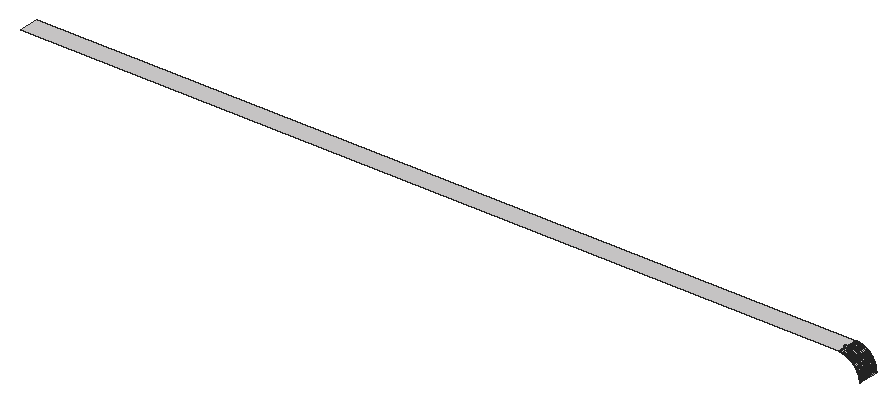
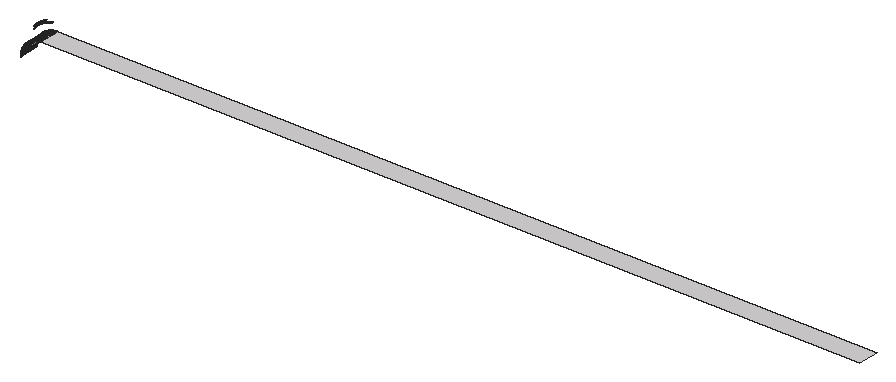
# SketchUp Ruby script. Lengths in inches.
U = 1.inch
M = Sketchup.active_model
def pt(a) = Geom::Point3d.new(a.map { |v| v * U })
def face(e, loops, mat)
  f = e.add_face(loops[0].map { |a| pt(a) })
  loops[1..].each { |l| e.add_face(l.map { |a| pt(a) }).erase! }
  f.material = f.back_material = mat if mat
  f
end
# faces: each face lists its corners as indices into pts; further lists are holes
def faces(e, pts, list, mat = nil) = list.each { |f| face(e, (f[0].is_a?(Array) ? f : [f]).map { |l| l.map { |i| pts[i] } }, mat) }
# xy, xz, yz: faces in a plane at the given z, y or x. An outline is a flat list of corners, or four numbers for a rectangle; further outlines are holes
def ring(l) = l.size == 4 ? [[l[0], l[1]], [l[2], l[1]], [l[2], l[3]], [l[0], l[3]]] : l.each_slice(2).to_a
def flat(e, list, mat, &to3) = list.each { |f| face(e, (f[0].is_a?(Array) ? f : [f]).map { |l| ring(l).map { |u, v| to3.(u, v) } }, mat) }
def xy(e, z, list, mat = nil) = flat(e, list, mat) { |x, y| [x, y, z] }
def xz(e, y, list, mat = nil) = flat(e, list, mat) { |x, z| [x, y, z] }
def yz(e, x, list, mat = nil) = flat(e, list, mat) { |y, z| [x, y, z] }
def lines(e, pts, list) = list.each { |a, b| e.add_line(pt(pts[a]), pt(pts[b])) }
# prism: a flat outline (further loops are holes) pulled along v
def prism(e, loops, v, mat = nil)
  f = face(e, loops, mat); d = Geom::Vector3d.new(v.map { |x| x * U })
  f.pushpull(f.normal.samedirection?(d) ? d.length : -d.length)
end
def box(e, o, s, mat = nil) = prism(e, [[o, [o[0] + s[0], o[1], o[2]], [o[0] + s[0], o[1] + s[1], o[2]], [o[0], o[1] + s[1], o[2]]]], [0, 0, s[2]], mat)
def at(x, y, z, deg = 0) = Geom::Transformation.translation(pt([x, y, z])) * Geom::Transformation.rotation(ORIGIN, Z_AXIS, deg.degrees)
def axes(o, x, y, z) = Geom::Transformation.new([*x, 0, *y, 0, *z, 0, *pt(o).to_a, 1])
def part(name) = M.definitions.add(name)
# library, detail: a bought-in or finely detailed component or shape, given as its bounding box
def library(name, o, s) = part(name).tap { |d| box(d.entities, o, s) }
def detail(e, o, s) = box(e.add_group.entities, o, s)
def put(e, d, t, mat = nil) = e.add_instance(d, t).tap { |i| i.material = mat if mat }
def group(e, t, mat = nil) = e.add_group.tap { |g| g.transformation = t; g.material = mat if mat }.entities
root = M.entities
M.materials.add("[Quartz Light Brown]").color = [215, 212, 212]
xy(root,95.96,[[504.94,38,505.04,50]],"[Quartz Light Brown]")
xy(root,95.98,[[504.66,38,504.75,50]],"[Quartz Light Brown]")
xy(root,95.99,[[504.375,38,504.47,50],[504.47,38,504.57,50]],"[Quartz Light Brown]")
xy(root,96,[[36,38,504,50],[504,38,504.09,50],[504.09,38,504.1875,50],[504.1875,38,504.28,50]],"[Quartz Light Brown]")
yz(root,515.96,[[38,84.94,50,85.04]],"[Quartz Light Brown]")
yz(root,515.98,[[38,84.66,50,84.75]],"[Quartz Light Brown]")
yz(root,515.99,[[38,84.375,50,84.47],[38,84.47,50,84.57]],"[Quartz Light Brown]")
yz(root,516,[[38,84,50,84.09],[38,84.09,50,84.1875],[38,84.1875,50,84.28]],"[Quartz Light Brown]")
p = [[516,38,84.28],[515.99,38,84.375],[515.99,50,84.375],[516,50,84.28],[515.99,38,84.57],[515.98,38,84.66],
  [515.98,50,84.66],[515.99,50,84.57],[515.97,38,84.85],[515.96,38,84.94],[515.96,50,84.94],[515.97,50,84.85],
  [515.98,38,84.75],[515.98,50,84.75],[515.96,38,85.04],[515.95,38,85.13],[515.95,50,85.13],[515.96,50,85.04],
  [515.9375,38,85.22],[515.9375,50,85.22],[515.93,38,85.32],[515.93,50,85.32],[515.92,38,85.41],[515.92,50,85.41],
  [515.91,38,85.5],[515.91,50,85.5],[515.89,38,85.6],[515.89,50,85.6],[515.88,38,85.69],[515.88,50,85.69],
  [515.87,38,85.78],[515.87,50,85.78],[515.85,38,85.88],[515.85,50,85.88],[515.84,38,85.97],[515.84,50,85.97],
  [515.82,38,86.0625],[515.82,50,86.0625],[515.8,38,86.16],[515.8,50,86.16],[515.79,38,86.25],[515.77,38,86.34],
  [515.77,50,86.34],[515.79,50,86.25],[515.75,38,86.43],[515.75,50,86.43],[515.73,38,86.53],[515.73,50,86.53],
  [515.71,38,86.62],[515.71,50,86.62],[515.69,38,86.71],[515.69,50,86.71],[515.67,38,86.8],[515.67,50,86.8],
  [515.65,38,86.89],[515.65,50,86.89],[515.62,38,86.98],[515.62,50,86.98],[515.6,38,87.08],[515.6,50,87.08],
  [515.57,38,87.17],[515.57,50,87.17],[515.55,38,87.26],[515.55,50,87.26],[515.52,38,87.35],[515.5,38,87.4375],
  [515.5,50,87.4375],[515.52,50,87.35],[515.47,38,87.53],[515.47,50,87.53],[515.44,38,87.62],[515.44,50,87.62],
  [515.41,38,87.71],[515.41,50,87.71],[515.38,38,87.8],[515.38,50,87.8],[515.35,38,87.89],[515.35,50,87.89],
  [515.32,38,87.98],[515.32,50,87.98],[515.29,38,88.06],[515.29,50,88.06],[515.26,38,88.15],[515.26,50,88.15],
  [515.23,38,88.24],[515.19,38,88.33],[515.19,50,88.33],[515.23,50,88.24],[515.16,38,88.42],[515.16,50,88.42],
  [515.12,38,88.5],[515.12,50,88.5],[515.09,38,88.59],[515.09,50,88.59],[515.05,38,88.68],[515.05,50,88.68],
  [515.01,38,88.77],[515.01,50,88.77],[514.98,38,88.85],[514.98,50,88.85],[514.9375,38,88.9375],[514.9,38,89.02],
  [514.9,50,89.02],[514.9375,50,88.9375],[514.86,38,89.11],[514.86,50,89.11],[514.82,38,89.19],[514.82,50,89.19],
  [514.78,38,89.28],[514.78,50,89.28],[514.73,38,89.36],[514.73,50,89.36],[514.69,38,89.45],[514.65,38,89.53],
  [514.65,50,89.53],[514.69,50,89.45],[514.61,38,89.62],[514.61,50,89.62],[514.5625,38,89.7],[514.5625,50,89.7],
  [514.52,38,89.78],[514.52,50,89.78],[514.47,38,89.86],[514.47,50,89.86],[514.42,38,89.95],[514.375,38,90.03],
  [514.375,50,90.03],[514.42,50,89.95],[514.33,38,90.11],[514.33,50,90.11],[514.28,38,90.1875],[514.28,50,90.1875],
  [514.23,38,90.27],[514.23,50,90.27],[514.18,38,90.35],[514.18,50,90.35],[514.13,38,90.43],[514.08,38,90.51],
  [514.08,50,90.51],[514.13,50,90.43],[514.03,38,90.59],[514.03,50,90.59],[513.98,38,90.67],[513.98,50,90.67],
  [513.92,38,90.75],[513.87,38,90.82],[513.87,50,90.82],[513.92,50,90.75],[513.82,38,90.9],[513.82,50,90.9],
  [513.76,38,90.98],[513.76,50,90.98],[513.71,38,91.05],[513.71,50,91.05],[513.65,38,91.13],[513.6,38,91.21],
  [513.6,50,91.21],[513.65,50,91.13],[513.54,38,91.28],[513.54,50,91.28],[513.48,38,91.35],[513.48,50,91.35],
  [513.42,38,91.43],[513.37,38,91.5],[513.37,50,91.5],[513.42,50,91.43],[513.31,38,91.58],[513.31,50,91.58],
  [513.25,38,91.65],[513.1875,38,91.72],[513.1875,50,91.72],[513.25,50,91.65],[513.125,38,91.79],[513.125,50,91.79],
  [513.0625,38,91.86],[513.0625,50,91.86],[513,38,91.9375],[512.9375,38,92.01],[512.9375,50,92.01],[513,50,91.9375],
  [512.875,38,92.08],[512.875,50,92.08],[512.8125,38,92.15],[512.75,38,92.21],[512.75,50,92.21],[512.8125,50,92.15],
  [512.68,38,92.28],[512.68,50,92.28],[512.62,38,92.35],[512.62,50,92.35],[512.55,38,92.42],[512.49,38,92.49],
  [512.49,50,92.49],[512.55,50,92.42],[512.42,38,92.55],[512.42,50,92.55],[512.35,38,92.62],[512.28,38,92.68],
  [512.28,50,92.68],[512.35,50,92.62],[512.21,38,92.75],[512.15,38,92.8125],[512.15,50,92.8125],[512.21,50,92.75],
  [512.08,38,92.875],[512.08,50,92.875],[512.01,38,92.9375],[511.9375,38,93],[511.9375,50,93],[512.01,50,92.9375],
  [511.86,38,93.0625],[511.86,50,93.0625],[511.79,38,93.125],[511.72,38,93.1875],[511.72,50,93.1875],[511.79,50,93.125],
  [511.65,38,93.25],[511.58,38,93.31],[511.58,50,93.31],[511.65,50,93.25],[511.5,38,93.37],[511.5,50,93.37],
  [511.43,38,93.42],[511.35,38,93.48],[511.35,50,93.48],[511.43,50,93.42],[516.87,39,93.51],[516.87,38,93.51],
  [516.94,38,93.4],[516.94,39,93.4],[511.28,38,93.54],[511.21,38,93.6],[511.21,50,93.6],[511.28,50,93.54],
  [516.79,39,93.61],[516.79,38,93.61],[511.13,38,93.65],[511.13,50,93.65],[516.72,39,93.71],[516.72,38,93.71],
  [511.05,38,93.71],[510.98,38,93.76],[510.98,50,93.76],[511.05,50,93.71],[516.64,39,93.81],[516.64,38,93.81],
  [510.9,38,93.82],[510.82,38,93.87],[510.82,50,93.87],[510.9,50,93.82],[516.56,39,93.91],[516.56,38,93.91],
  [510.75,38,93.92],[510.67,38,93.98],[510.67,50,93.98],[510.75,50,93.92],[516.49,39,94],[516.49,38,94],
  [510.59,38,94.03],[510.51,38,94.08],[510.51,50,94.08],[510.59,50,94.03],[516.41,39,94.1],[516.41,38,94.1],
  [510.43,38,94.13],[510.35,38,94.18],[510.35,50,94.18],[510.43,50,94.13],[516.33,39,94.2],[516.33,38,94.2],
  [510.27,38,94.23],[510.1875,38,94.28],[510.1875,50,94.28],[510.27,50,94.23],[516.25,39,94.3],[516.25,38,94.3],
  [510.11,38,94.33],[510.03,38,94.375],[510.03,50,94.375],[510.11,50,94.33],[516.17,39,94.39],[516.17,38,94.39],
  [509.95,38,94.42],[509.86,38,94.47],[509.86,50,94.47],[509.95,50,94.42],[516.08,39,94.49],[516.08,38,94.49],
  [509.78,38,94.52],[509.7,38,94.5625],[509.7,50,94.5625],[509.78,50,94.52],[516,39,94.58],[516,38,94.58],
  [509.53,38,94.65],[509.45,38,94.69],[509.45,50,94.69],[509.53,50,94.65],[509.62,38,94.61],[509.62,50,94.61],
  [515.92,39,94.67],[515.92,38,94.67],[509.36,38,94.73],[509.28,38,94.78],[509.28,50,94.78],[509.36,50,94.73],
  [515.83,39,94.77],[515.83,38,94.77],[509.19,38,94.82],[509.11,38,94.86],[509.11,50,94.86],[509.19,50,94.82],
  [515.75,39,94.86],[515.75,38,94.86],[508.9375,38,94.9375],[508.85,38,94.98],[508.85,50,94.98],[508.9375,50,94.9375],
  [509.02,38,94.9],[509.02,50,94.9],[515.66,39,94.95],[515.66,38,94.95],[508.77,38,95.01],[508.68,38,95.05],
  [508.68,50,95.05],[508.77,50,95.01],[515.49,39,95.13],[515.49,38,95.13],[515.58,38,95.04],[515.58,39,95.04],
  [516.84,38,95.14],[516.84,39,95.14],[516.93,39,95.04],[516.93,38,95.04],[508.5,38,95.12],[508.42,38,95.16],
  [508.42,50,95.16],[508.5,50,95.12],[508.59,38,95.09],[508.59,50,95.09],[515.4,39,95.22],[515.4,38,95.22],
  [516.75,38,95.24],[516.75,39,95.24],[508.24,38,95.23],[508.15,38,95.26],[508.15,50,95.26],[508.24,50,95.23],
  [508.33,38,95.19],[508.33,50,95.19],[515.3125,39,95.3125],[515.3125,38,95.3125],[516.66,38,95.34],[516.66,39,95.34],
  [507.98,38,95.32],[507.89,38,95.35],[507.89,50,95.35],[507.98,50,95.32],[508.06,38,95.29],[508.06,50,95.29],
  [515.22,39,95.4],[515.22,38,95.4],[516.57,38,95.44],[516.57,39,95.44],[507.62,38,95.44],[507.53,38,95.47],
  [507.53,50,95.47],[507.62,50,95.44],[507.71,38,95.41],[507.71,50,95.41],[507.8,38,95.38],[507.8,50,95.38],
  [515.13,39,95.49],[515.13,38,95.49],[516.48,38,95.54],[516.48,39,95.54],[507.26,38,95.55],[507.17,38,95.57],
  [507.17,50,95.57],[507.26,50,95.55],[507.35,38,95.52],[507.35,50,95.52],[507.4375,38,95.5],[507.4375,50,95.5],
  [515.04,39,95.58],[515.04,38,95.58],[516.39,38,95.64],[516.39,39,95.64],[506.89,38,95.65],[506.8,38,95.67],
  [506.8,50,95.67],[506.89,50,95.65],[506.98,38,95.62],[506.98,50,95.62],[507.08,38,95.6],[507.08,50,95.6],
  [514.95,39,95.66],[514.95,38,95.66],[516.3,38,95.73],[516.3,39,95.73],[506.53,38,95.73],[506.43,38,95.75],
  [506.43,50,95.75],[506.53,50,95.73],[506.62,38,95.71],[506.62,50,95.71],[506.71,38,95.69],[506.71,50,95.69],
  [514.77,39,95.83],[514.77,38,95.83],[514.86,38,95.75],[514.86,39,95.75],[516.21,38,95.83],[516.21,39,95.83],
  [505.97,38,95.84],[505.88,38,95.85],[505.88,50,95.85],[505.97,50,95.84],[506.0625,38,95.82],[506.0625,50,95.82],
  [506.16,38,95.8],[506.16,50,95.8],[506.25,38,95.79],[506.25,50,95.79],[506.34,38,95.77],[506.34,50,95.77],
  [514.67,39,95.92],[514.67,38,95.92],[516.11,38,95.93],[516.11,39,95.93],[505.13,38,95.95],[505.04,38,95.96],
  [505.04,50,95.96],[505.13,50,95.95],[505.22,38,95.9375],[505.22,50,95.9375],[505.32,38,95.93],[505.32,50,95.93],
  [505.41,38,95.92],[505.41,50,95.92],[505.5,38,95.91],[505.5,50,95.91],[505.6,38,95.89],[505.6,50,95.89],
  [505.69,38,95.88],[505.69,50,95.88],[505.78,38,95.87],[505.78,50,95.87],[514.58,39,96],[514.58,38,96],
  [516.02,38,96.02],[516.02,39,96.02],[504.375,38,95.99],[504.28,38,96],[504.28,50,96],[504.375,50,95.99],
  [504.66,38,95.98],[504.57,38,95.99],[504.57,50,95.99],[504.66,50,95.98],[504.85,38,95.97],[504.75,38,95.98],
  [504.75,50,95.98],[504.85,50,95.97],[504.94,38,95.96],[504.94,50,95.96],[514.49,39,96.08],[514.49,38,96.08],
  [515.93,38,96.11],[515.93,39,96.11],[514.39,39,96.17],[514.39,38,96.17],[515.83,38,96.21],[515.83,39,96.21],
  [514.2,39,96.33],[514.2,38,96.33],[514.3,38,96.25],[514.3,39,96.25],[515.73,38,96.3],[515.73,39,96.3],
  [514.1,39,96.41],[514.1,38,96.41],[515.64,38,96.39],[515.64,39,96.39],[514,39,96.49],[514,38,96.49],
  [515.54,38,96.48],[515.54,39,96.48],[513.91,39,96.56],[513.91,38,96.56],[515.44,38,96.57],[515.44,39,96.57],
  [513.71,39,96.72],[513.71,38,96.72],[513.81,38,96.64],[513.81,39,96.64],[515.34,38,96.66],[515.34,39,96.66],
  [513.61,39,96.79],[513.61,38,96.79],[515.24,38,96.75],[515.24,39,96.75],[513.51,39,96.87],[513.51,38,96.87],
  [515.04,38,96.93],[515.04,39,96.93],[515.14,39,96.84],[515.14,38,96.84],[513.3,39,97.02],[513.3,38,97.02],
  [513.4,38,96.94],[513.4,39,96.94],[514.9375,38,97.01],[514.9375,39,97.01],[513.2,39,97.09],[513.2,38,97.09],
  [514.84,38,97.1],[514.84,39,97.1],[513.1,39,97.16],[513.1,38,97.16],[514.73,38,97.18],[514.73,39,97.18],
  [512.89,39,97.3],[512.89,38,97.3],[512.99,38,97.23],[512.99,39,97.23],[514.63,38,97.27],[514.63,39,97.27],
  [512.78,39,97.37],[512.78,38,97.37],[514.52,38,97.35],[514.52,39,97.35],[512.57,39,97.51],[512.57,38,97.51],
  [512.68,38,97.44],[512.68,39,97.44],[514.3125,38,97.51],[514.3125,39,97.51],[514.42,39,97.43],[514.42,38,97.43],
  [512.47,39,97.58],[512.47,38,97.58],[514.21,38,97.59],[514.21,39,97.59],[512.25,39,97.71],[512.25,38,97.71],
  [512.36,38,97.64],[512.36,39,97.64],[514.1,38,97.67],[514.1,39,97.67],[512.14,39,97.77],[512.14,38,97.77],
  [513.99,38,97.75],[513.99,39,97.75],[511.93,39,97.9],[511.93,38,97.9],[512.04,38,97.84],[512.04,39,97.84],
  [513.78,38,97.91],[513.78,39,97.91],[513.88,39,97.83],[513.88,38,97.83],[511.82,39,97.96],[511.82,38,97.96],
  [513.67,38,97.98],[513.67,39,97.98],[511.6,39,98.08],[511.6,38,98.08],[511.71,38,98.02],[511.71,39,98.02],
  [513.56,38,98.06],[513.56,39,98.06],[511.375,39,98.2],[511.375,38,98.2],[511.49,38,98.14],[511.49,39,98.14],
  [513.33,38,98.21],[513.33,39,98.21],[513.44,39,98.13],[513.44,38,98.13],[511.26,39,98.26],[511.26,38,98.26],
  [513.22,38,98.28],[513.22,39,98.28],[511.04,39,98.37],[511.04,38,98.37],[511.15,38,98.3125],[511.15,39,98.3125],
  [513.11,38,98.35],[513.11,39,98.35],[510.8125,39,98.48],[510.8125,38,98.48],[510.93,38,98.42],[510.93,39,98.42],
  [512.88,38,98.49],[512.88,39,98.49],[513,39,98.42],[513,38,98.42],[510.58,39,98.58],[510.58,38,98.58],
  [510.7,38,98.53],[510.7,39,98.53],[512.77,38,98.5625],[512.77,39,98.5625],[510.35,39,98.68],[510.35,38,98.68],
  [510.47,38,98.63],[510.47,39,98.63],[512.54,38,98.7],[512.54,39,98.7],[512.65,39,98.63],[512.65,38,98.63],
  [510.12,39,98.78],[510.12,38,98.78],[510.24,38,98.73],[510.24,39,98.73],[512.42,38,98.77],[512.42,39,98.77],
  [509.89,39,98.875],[509.89,38,98.875],[510.01,38,98.83],[510.01,39,98.83],[512.19,38,98.9],[512.19,39,98.9],
  [512.31,39,98.83],[512.31,38,98.83],[509.66,39,98.97],[509.66,38,98.97],[509.77,38,98.92],[509.77,39,98.92],
  [512.07,38,98.96],[512.07,39,98.96],[509.42,39,99.05],[509.42,38,99.05],[509.54,38,99.01],[509.54,39,99.01],
  [511.84,38,99.09],[511.84,39,99.09],[511.95,39,99.02],[511.95,38,99.02],[509.0625,39,99.18],[509.0625,38,99.18],
  [509.18,38,99.14],[509.18,39,99.14],[509.3,38,99.1],[509.3,39,99.1],[511.6,38,99.21],[511.6,39,99.21],
  [511.72,39,99.15],[511.72,38,99.15],[508.82,39,99.26],[508.82,38,99.26],[508.94,38,99.22],[508.94,39,99.22],
  [511.48,38,99.27],[511.48,39,99.27],[508.46,39,99.36],[508.46,38,99.36],[508.58,38,99.33],[508.58,39,99.33],
  [508.7,38,99.29],[508.7,39,99.29],[511.24,38,99.38],[511.24,39,99.38],[511.36,39,99.32],[511.36,38,99.32],
  [508.1,39,99.47],[508.1,38,99.47],[508.22,38,99.43],[508.22,39,99.43],[508.34,38,99.4],[508.34,39,99.4],
  [511,38,99.49],[511,39,99.49],[511.12,39,99.4375],[511.12,38,99.4375],[507.74,39,99.56],[507.74,38,99.56],
  [507.86,38,99.53],[507.86,39,99.53],[507.98,38,99.5],[507.98,39,99.5],[510.75,38,99.6],[510.75,39,99.6],
  [510.875,39,99.55],[510.875,38,99.55],[507.24,39,99.67],[507.24,38,99.67],[507.37,38,99.64],[507.37,39,99.64],
  [507.49,38,99.61],[507.49,39,99.61],[507.61,38,99.59],[507.61,39,99.59],[510.63,38,99.65],[510.63,39,99.65],
  [506.75,39,99.76],[506.75,38,99.76],[506.875,38,99.74],[506.875,39,99.74],[507,38,99.72],[507,39,99.72],
  [507.12,38,99.69],[507.12,39,99.69],[510.38,38,99.76],[510.38,39,99.76],[510.51,39,99.71],[510.51,38,99.71],
  [510.26,38,99.81],[510.26,39,99.81]]
faces(root,p,[[0,1,2,3],[4,5,6,7],[8,9,10,11],[12,8,11,13],[14,15,16,17],[15,18,19,16],[18,20,21,19],[20,22,23,21],
  [22,24,25,23],[24,26,27,25],[26,28,29,27],[28,30,31,29],[30,32,33,31],[32,34,35,33],[34,36,37,35],[36,38,39,37],
  [40,41,42,43],[38,40,43,39],[41,44,45,42],[44,46,47,45],[46,48,49,47],[48,50,51,49],[50,52,53,51],[52,54,55,53],
  [54,56,57,55],[56,58,59,57],[58,60,61,59],[60,62,63,61],[64,65,66,67],[62,64,67,63],[65,68,69,66],[68,70,71,69],
  [70,72,73,71],[72,74,75,73],[74,76,77,75],[76,78,79,77],[78,80,81,79],[80,82,83,81],[84,85,86,87],[82,84,87,83],
  [85,88,89,86],[88,90,91,89],[90,92,93,91],[92,94,95,93],[94,96,97,95],[96,98,99,97],[100,101,102,103],[98,100,103,99],
  [101,104,105,102],[104,106,107,105],[106,108,109,107],[108,110,111,109],[112,113,114,115],[110,112,115,111],[113,116,117,114],[116,118,119,117],
  [118,120,121,119],[120,122,123,121],[124,125,126,127],[122,124,127,123],[125,128,129,126],[128,130,131,129],[130,132,133,131],[132,134,135,133],
  [136,137,138,139],[134,136,139,135],[137,140,141,138],[140,142,143,141],[144,145,146,147],[142,144,147,143],[145,148,149,146],[148,150,151,149],
  [150,152,153,151],[154,155,156,157],[152,154,157,153],[155,158,159,156],[158,160,161,159],[162,163,164,165],[160,162,165,161],[163,166,167,164],
  [168,169,170,171],[166,168,171,167],[169,172,173,170],[172,174,175,173],[176,177,178,179],[174,176,179,175],[177,180,181,178],[182,183,184,185],
  [180,182,185,181],[183,186,187,184],[186,188,189,187],[190,191,192,193],[188,190,193,189],[191,194,195,192],[196,197,198,199],[194,196,199,195],
  [200,201,202,203],[197,200,203,198],[201,204,205,202],[206,207,208,209],[204,206,209,205],[207,210,211,208],[212,213,214,215],[210,212,215,211],
  [216,217,218,219],[213,216,219,214],[217,220,221,218],[222,223,224,225],[220,222,225,221],[226,227,228,229],[230,231,232,233],[223,230,233,224],
  [234,235,227,226],[231,236,237,232],[238,239,235,234],[240,241,242,243],[236,240,243,237],[244,245,239,238],[246,247,248,249],[241,246,249,242],
  [250,251,245,244],[252,253,254,255],[247,252,255,248],[256,257,251,250],[258,259,260,261],[253,258,261,254],[262,263,257,256],[264,265,266,267],
  [259,264,267,260],[268,269,263,262],[270,271,272,273],[265,270,273,266],[274,275,269,268],[276,277,278,279],[271,276,279,272],[280,281,275,274],
  [282,283,284,285],[277,282,285,278],[286,287,281,280],[288,289,290,291],[283,288,291,284],[292,293,287,286],[294,295,296,297],[298,294,297,299],
  [289,298,299,290],[300,301,293,292],[302,303,304,305],[295,302,305,296],[306,307,301,300],[308,309,310,311],[303,308,311,304],[312,313,307,306],
  [314,315,316,317],[318,314,317,319],[309,318,319,310],[320,321,313,312],[322,323,324,325],[315,322,325,316],[326,327,328,329],[329,328,321,320],
  [330,331,332,333],[334,335,336,337],[338,334,337,339],[323,338,339,324],[340,341,327,326],[342,343,331,330],[344,345,346,347],[348,344,347,349],
  [335,348,349,336],[350,351,341,340],[352,353,343,342],[354,355,356,357],[358,354,357,359],[345,358,359,346],[360,361,351,350],[362,363,353,352],
  [364,365,366,367],[368,364,367,369],[370,368,369,371],[355,370,371,356],[372,373,361,360],[374,375,363,362],[376,377,378,379],[380,376,379,381],
  [382,380,381,383],[365,382,383,366],[384,385,373,372],[386,387,375,374],[388,389,390,391],[392,388,391,393],[394,392,393,395],[377,394,395,378],
  [396,397,385,384],[398,399,387,386],[400,401,402,403],[404,400,403,405],[406,404,405,407],[389,406,407,390],[408,409,410,411],[411,410,397,396],
  [412,413,399,398],[414,415,416,417],[418,414,417,419],[420,418,419,421],[422,420,421,423],[424,422,423,425],[401,424,425,402],[426,427,409,408],
  [428,429,413,412],[430,431,432,433],[434,430,433,435],[436,434,435,437],[438,436,437,439],[440,438,439,441],[442,440,441,443],[444,442,443,445],
  [446,444,445,447],[415,446,447,416],[448,449,427,426],[450,451,429,428],[452,453,454,455],[456,457,458,459],[460,461,462,463],[464,460,463,465],
  [466,467,449,448],[468,469,451,450],[470,471,467,466],[472,473,469,468],[474,475,476,477],[477,476,471,470],[478,479,473,472],[480,481,475,474],
  [482,483,479,478],[484,485,481,480],[486,487,483,482],[488,489,485,484],[490,491,487,486],[492,493,494,495],[495,494,489,488],[496,497,491,490],
  [498,499,493,492],[500,501,497,496],[502,503,499,498],[504,505,506,507],[507,506,501,500],[508,509,510,511],[511,510,503,502],[512,513,505,504],
  [514,515,509,508],[516,517,513,512],[518,519,515,514],[520,521,517,516],[522,523,524,525],[525,524,519,518],[526,527,521,520],[528,529,523,522],
  [530,531,527,526],[532,533,534,535],[535,534,529,528],[536,537,538,539],[539,538,531,530],[540,541,533,532],[542,543,537,536],[544,545,546,547],
  [547,546,541,540],[548,549,543,542],[550,551,545,544],[552,553,549,548],[554,555,556,557],[557,556,551,550],[558,559,560,561],[561,560,553,552],
  [562,563,555,554],[564,565,559,558],[566,567,568,569],[569,568,563,562],[570,571,565,564],[572,573,574,575],[575,574,567,566],[576,577,578,579],
  [579,578,571,570],[580,581,573,572],[582,583,577,576],[584,585,586,587],[587,586,581,580],[588,589,583,582],[590,591,592,593],[593,592,585,584],
  [594,595,596,597],[597,596,589,588],[598,599,600,601],[601,600,591,590],[602,603,595,594],[604,605,606,607],[607,606,599,598],[608,609,610,611],
  [611,610,603,602],[612,613,614,615],[615,614,605,604],[616,617,609,608],[618,619,620,621],[621,620,613,612],[622,623,624,625],[625,624,617,616],
  [626,627,628,629],[629,628,619,618],[630,631,623,622],[632,633,634,635],[635,634,627,626],[636,637,638,639],[639,638,631,630],[640,641,642,643],
  [643,642,644,645],[645,644,633,632],[646,647,648,649],[649,648,637,636],[650,651,652,653],[653,652,641,640],[654,655,647,646],[656,657,658,659],
  [659,658,660,661],[661,660,651,650],[662,663,664,665],[665,664,655,654],[666,667,668,669],[669,668,670,671],[671,670,657,656],[672,673,674,675],
  [675,674,663,662],[676,677,678,679],[679,678,680,681],[681,680,667,666],[682,683,684,685],[685,684,673,672],[686,687,688,689],[689,688,690,691],
  [691,690,692,693],[693,692,677,676],[694,695,683,682],[696,697,698,699],[699,698,700,701],[701,700,702,703],[703,702,687,686],[704,705,706,707],
  [707,706,695,694],[708,709,705,704]],"[Quartz Light Brown]")
